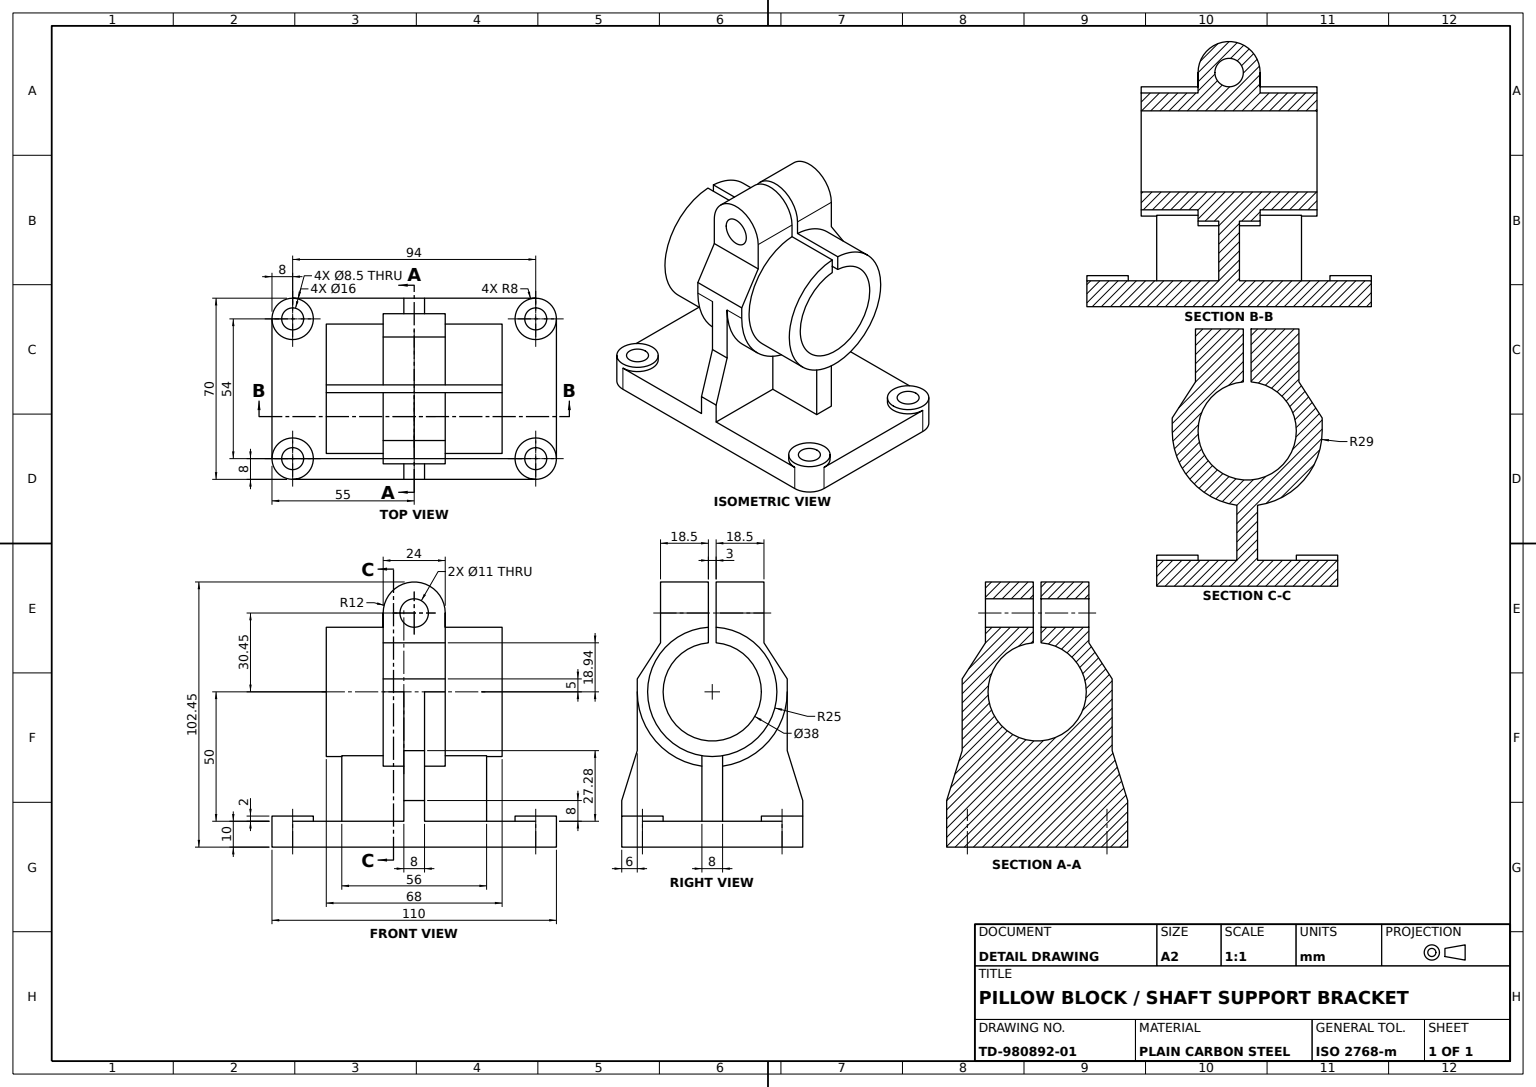
solid
v1 (47,-48,35)
v2 (47,-48,19)
e1 v1 v2 CIRCLE(AX(P(47,-48,27),D(0,1,0),D(0,0,1)),8)
e2 v2 v1 CIRCLE(AX(P(47,-48,27),D(0,1,0),D(0,0,1)),8)
v3 (47,-48,22.75)
v4 (47,-48,31.25)
e3 v3 v4 CIRCLE(AX(P(47,-48,27),D(0,1,0),D(0,0,1)),4.25)
e4 v4 v3 CIRCLE(AX(P(47,-48,27),D(0,1,0),D(0,0,1)),4.25)
face PLANE(AX(P(47,-48,27),D(0,1,0),D(0,0,1))) [e1 e2] [-e3 -e4]
v5 (-34,0,-19)
v6 (-34,0,19)
e5 v5 v6 CIRCLE(AX(P(-34,0,0),D(-1,0,0),D(0,0,1)),19)
v7 (34,0,19)
e6 v7 v6 LINE
v8 (34,0,-19)
e7 v8 v7 CIRCLE(AX(P(34,0,0),D(-1,0,0),D(0,0,1)),19)
e8 v8 v5 LINE
face CYL(AX(P(34,0,0),D(-1,0,0),D(0,0,1)),19) rev [e5 -e6 -e7 e8]
v9 (-12,0,-25)
v10 (-34,0,-25)
e9 v9 v10 LINE
v11 (-34,24.954959,-1.5)
e10 v10 v11 CIRCLE(AX(P(-34,0,0),D(1,0,0),D(0,0,1)),25)
v12 (-12,24.954959,-1.5)
e11 v12 v11 LINE
e12 v12 v9 CIRCLE(AX(P(-12,0,0),D(-1,0,0),D(0,0,1)),25)
face CYL(AX(P(34,0,0),D(-1,0,0),D(0,0,1)),25) [e9 e10 -e11 e12]
v13 (-4,-42,35)
v14 (-4,-50,35)
e13 v13 v14 LINE
v15 (-4,-22.719786,29)
e14 v15 v13 LINE
v16 (-4,0,29)
e15 v16 v15 LINE
v17 (-4,-28.722813,4)
e16 v16 v17 CIRCLE(AX(P(-4,0,0),D(1,0,0),D(0,0,-1)),29)
v18 (-4,-50,4)
e17 v17 v18 LINE
e18 v18 v14 LINE
face PLANE(AX(P(-4,-8.77252,0),D(1,0,0),D(0,0,-1))) rev [-e13 -e14 -e15 e16 e17 e18]
v19 (34,0,25)
v20 (12,0,25)
e19 v19 v20 LINE
v21 (34,24.954959,1.5)
e20 v21 v19 CIRCLE(AX(P(34,0,0),D(1,0,0),D(0,0,1)),25)
v22 (12,24.954959,1.5)
e21 v21 v22 LINE
e22 v20 v22 CIRCLE(AX(P(12,0,0),D(-1,0,0),D(0,0,1)),25)
face CYL(AX(P(34,0,0),D(-1,0,0),D(0,0,1)),25) [-e19 -e20 e21 -e22]
v23 (-4,-42,-35)
v24 (-4,-50,-35)
e23 v23 v24 LINE
v25 (-4,-50,-4)
e24 v24 v25 LINE
v26 (-4,-28.722813,-4)
e25 v25 v26 LINE
v27 (-4,0,-29)
e26 v27 v26 CIRCLE(AX(P(-4,0,0),D(-1,0,0),D(0,0,-1)),29)
v28 (-4,-22.719786,-29)
e27 v27 v28 LINE
e28 v28 v23 LINE
face PLANE(AX(P(-4,-8.77252,0),D(1,0,0),D(0,0,-1))) rev [e23 e24 e25 -e26 e27 e28]
v29 (12,24.954959,-1.5)
v30 (12,30.454959,-1.5)
e29 v29 v30 LINE
v31 (-12,30.454959,-1.5)
e30 v30 v31 CIRCLE(AX(P(0,30.454959,-1.5),D(0,0,1),D(1,0,0)),12)
e31 v31 v12 LINE
v32 (-34,18.940697,-1.5)
e32 v11 v32 LINE
v33 (34,18.940697,-1.5)
e33 v33 v32 LINE
v34 (34,24.954959,-1.5)
e34 v34 v33 LINE
e35 v34 v29 LINE
v35 (5.5,30.454959,-1.5)
v36 (-5.5,30.454959,-1.5)
e36 v35 v36 CIRCLE(AX(P(0,30.454959,-1.5),D(0,0,1),D(1,0,0)),5.5)
e37 v36 v35 CIRCLE(AX(P(0,30.454959,-1.5),D(0,0,1),D(1,0,0)),5.5)
face PLANE(AX(P(34,18.940697,-1.5),D(0,0,-1),D(-1,0,0))) rev [e29 e30 e31 e11 e32 -e33 -e34 e35] [-e36 -e37]
v37 (47,-60,-22.75)
v38 (47,-48,-22.75)
e38 v37 v38 LINE
v39 (47,-60,-31.25)
e39 v39 v37 CIRCLE(AX(P(47,-60,-27),D(0,1,0),D(0,0,-1)),4.25)
v40 (47,-48,-31.25)
e40 v39 v40 LINE
e41 v40 v38 CIRCLE(AX(P(47,-48,-27),D(0,1,0),D(0,0,1)),4.25)
face CYL(AX(P(47,-60.001,-27),D(0,1,0),D(0,0,1)),4.25) rev [-e38 -e39 e40 e41]
v41 (55,-60,27)
v42 (47,-60,35)
e42 v41 v42 CIRCLE(AX(P(47,-60,27),D(0,-1,0),D(0,0,-1)),8)
v43 (55,-50,27)
e43 v41 v43 LINE
v44 (47,-50,19)
e44 v43 v44 CIRCLE(AX(P(47,-50,27),D(0,1,0),D(0,0,1)),8)
e45 v44 v2 LINE
v45 (47,-50,35)
e46 v45 v1 LINE
e47 v42 v45 LINE
face CYL(AX(P(47,-60,27),D(0,1,0),D(0,0,1)),8) [-e42 e43 e44 e45 -e1 -e46 -e47]
v46 (-47,-60,-31.25)
v47 (-47,-48,-31.25)
e48 v46 v47 LINE
v48 (-47,-60,-22.75)
e49 v48 v46 CIRCLE(AX(P(-47,-60,-27),D(0,1,0),D(0,0,-1)),4.25)
v49 (-47,-48,-22.75)
e50 v48 v49 LINE
e51 v49 v47 CIRCLE(AX(P(-47,-48,-27),D(0,1,0),D(0,0,1)),4.25)
face CYL(AX(P(-47,-60.001,-27),D(0,1,0),D(0,0,1)),4.25) rev [-e48 -e49 e50 e51]
v50 (12,-28.722813,4)
v51 (4,-28.722813,4)
e52 v50 v51 LINE
v52 (12,0,29)
e53 v52 v50 CIRCLE(AX(P(12,0,0),D(1,0,0),D(0,0,-1)),29)
v53 (4,0,29)
e54 v52 v53 LINE
e55 v53 v51 CIRCLE(AX(P(4,0,0),D(1,0,0),D(0,0,-1)),29)
face CYL(AX(P(12,0,0),D(-1,0,0),D(0,0,1)),29) [-e52 -e53 e54 e55]
v54 (-12,0,-29)
v55 (-12,-28.722813,-4)
e56 v54 v55 CIRCLE(AX(P(-12,0,0),D(-1,0,0),D(0,0,1)),29)
v56 (-12,-24.677925,-4)
e57 v55 v56 LINE
e58 v9 v56 CIRCLE(AX(P(-12,0,0),D(-1,0,0),D(0,0,1)),25)
v57 (-12,30.454959,-20)
e59 v57 v31 LINE
v58 (-12,18.940697,-20)
e60 v57 v58 LINE
v59 (-12,5,-29)
e61 v58 v59 LINE
e62 v59 v54 LINE
face PLANE(AX(P(-12,30.454959,-20),D(-1,0,0),D(0,0,1))) [e56 e57 -e58 -e12 -e31 -e59 e60 e61 e62]
v60 (-34,24.954959,1.5)
v61 (-34,0,25)
e63 v60 v61 CIRCLE(AX(P(-34,0,0),D(1,0,0),D(0,0,1)),25)
v62 (-12,0,25)
e64 v62 v61 LINE
v63 (-12,24.954959,1.5)
e65 v63 v62 CIRCLE(AX(P(-12,0,0),D(1,0,0),D(0,0,-1)),25)
e66 v63 v60 LINE
face CYL(AX(P(34,0,0),D(-1,0,0),D(0,0,1)),25) [e63 -e64 -e65 e66]
v64 (-47,-60,31.25)
v65 (-47,-48,31.25)
e67 v64 v65 LINE
v66 (-47,-60,22.75)
e68 v66 v64 CIRCLE(AX(P(-47,-60,27),D(0,1,0),D(0,0,-1)),4.25)
v67 (-47,-48,22.75)
e69 v66 v67 LINE
e70 v67 v65 CIRCLE(AX(P(-47,-48,27),D(0,1,0),D(0,0,1)),4.25)
face CYL(AX(P(-47,-60.001,27),D(0,1,0),D(0,0,1)),4.25) rev [-e67 -e68 e69 e70]
v68 (-5.5,30.454959,-20)
e71 v68 v36 LINE
v69 (5.5,30.454959,-20)
e72 v69 v68 CIRCLE(AX(P(0,30.454959,-20),D(0,0,1),D(1,0,0)),5.5)
e73 v69 v35 LINE
face CYL(AX(P(0,30.454959,-20),D(0,0,1),D(1,0,0)),5.5) rev [-e71 -e72 e73 e36]
v70 (47,-50,-35)
v71 (47,-50,-19)
e74 v70 v71 CIRCLE(AX(P(47,-50,-27),D(0,1,0),D(0,0,1)),8)
v72 (47,-48,-19)
e75 v71 v72 LINE
v73 (47,-48,-35)
e76 v73 v72 CIRCLE(AX(P(47,-48,-27),D(0,1,0),D(0,0,1)),8)
e77 v70 v73 LINE
face CYL(AX(P(47,-60,-27),D(0,1,0),D(0,0,1)),8) [e74 e75 -e76 -e77]
v74 (-12,-24.677925,4)
v75 (-28,-24.677925,4)
e78 v74 v75 LINE
v76 (-28,-50,4)
e79 v75 v76 LINE
e80 v18 v76 LINE
v77 (-12,-28.722813,4)
e81 v17 v77 LINE
e82 v77 v74 LINE
face PLANE(AX(P(28,-50,4),D(0,0,-1),D(0,1,0))) rev [e78 e79 -e80 -e17 e81 e82]
v78 (-47,-48,35)
v79 (-47,-48,19)
e83 v78 v79 CIRCLE(AX(P(-47,-48,27),D(0,1,0),D(0,0,1)),8)
v80 (-47,-50,35)
e84 v80 v78 LINE
v81 (-47,-50,19)
e85 v80 v81 CIRCLE(AX(P(-47,-50,27),D(0,1,0),D(0,0,1)),8)
e86 v81 v79 LINE
face CYL(AX(P(-47,-60,27),D(0,1,0),D(0,0,1)),8) [-e83 -e84 e85 e86]
v82 (4,-50,35)
e87 v45 v82 LINE
v83 (4,-42,35)
e88 v83 v82 LINE
e89 v13 v83 LINE
e90 v14 v80 LINE
v84 (-47,-60,35)
e91 v84 v80 LINE
e92 v42 v84 LINE
face PLANE(AX(P(47,-60,35),D(0,0,-1),D(-1,0,0))) rev [e87 -e88 -e89 e13 e90 -e91 -e92 e47]
e93 v46 v48 CIRCLE(AX(P(-47,-60,-27),D(0,1,0),D(0,0,-1)),4.25)
e94 v47 v49 CIRCLE(AX(P(-47,-48,-27),D(0,1,0),D(0,0,1)),4.25)
face CYL(AX(P(-47,-60.001,-27),D(0,1,0),D(0,0,1)),4.25) rev [-e50 -e93 e48 e94]
v85 (4,-22.719786,-29)
e95 v28 v85 LINE
v86 (4,-42,-35)
e96 v85 v86 LINE
e97 v23 v86 LINE
face PLANE(AX(P(0,-22.719786,-29),D(0,-0.297143819,0.954832735),D(0,-0.954832735,-0.297143819))) rev [-e28 e95 e96 -e97]
v87 (34,0,-25)
e98 v19 v87 CIRCLE(AX(P(34,0,0),D(1,0,0),D(0,0,1)),25)
e99 v87 v34 CIRCLE(AX(P(34,0,0),D(1,0,0),D(0,0,1)),25)
e100 v33 v8 CIRCLE(AX(P(34,0,0),D(-1,0,0),D(0,0,1)),19)
v88 (34,18.940697,1.5)
e101 v7 v88 CIRCLE(AX(P(34,0,0),D(-1,0,0),D(0,0,1)),19)
e102 v88 v21 LINE
face PLANE(AX(P(34,0,0),D(-1,0,0),D(0,0,1))) rev [e20 e98 e99 e34 e100 e7 e101 e102]
e103 v44 v45 CIRCLE(AX(P(47,-50,27),D(0,1,0),D(0,0,1)),8)
face CYL(AX(P(47,-60,27),D(0,1,0),D(0,0,1)),8) [-e45 e103 e46 -e2]
v89 (4,-50,-35)
e104 v86 v89 LINE
e105 v89 v70 LINE
v90 (47,-60,-35)
e106 v90 v70 LINE
v91 (-47,-60,-35)
e107 v91 v90 LINE
v92 (-47,-50,-35)
e108 v91 v92 LINE
e109 v92 v24 LINE
face PLANE(AX(P(47,-60,-35),D(0,0,1),D(1,0,0))) rev [e104 e105 -e106 -e107 e108 e109 -e23 e97]
e110 v65 v67 CIRCLE(AX(P(-47,-48,27),D(0,1,0),D(0,0,1)),4.25)
e111 v64 v66 CIRCLE(AX(P(-47,-60,27),D(0,1,0),D(0,0,-1)),4.25)
face CYL(AX(P(-47,-60.001,27),D(0,1,0),D(0,0,1)),4.25) rev [e110 -e69 -e111 e67]
v93 (-28,-24.677925,-4)
e112 v56 v93 LINE
e113 v93 v75 CIRCLE(AX(P(-28,0,0),D(-1,0,0),D(0,0,-1)),25)
e114 v62 v74 CIRCLE(AX(P(-12,0,0),D(1,0,0),D(0,0,-1)),25)
e115 v61 v10 CIRCLE(AX(P(-34,0,0),D(1,0,0),D(0,0,1)),25)
face CYL(AX(P(34,0,0),D(-1,0,0),D(0,0,1)),25) [-e9 e58 e112 e113 -e78 -e114 e64 e115]
e116 v68 v69 CIRCLE(AX(P(0,30.454959,-20),D(0,0,1),D(1,0,0)),5.5)
face CYL(AX(P(0,30.454959,-20),D(0,0,1),D(1,0,0)),5.5) rev [-e73 -e116 e71 e37]
v94 (4,-22.719786,29)
e117 v15 v94 LINE
e118 v94 v83 LINE
face PLANE(AX(P(0,-22.719786,29),D(0,0.297143819,0.954832735),D(0,-0.954832735,0.297143819))) [-e117 e14 e89 -e118]
v95 (12,-28.722813,-4)
v96 (12,-24.677925,-4)
e119 v95 v96 LINE
v97 (12,0,-29)
e120 v97 v95 CIRCLE(AX(P(12,0,0),D(-1,0,0),D(0,0,1)),29)
v98 (12,5,-29)
e121 v98 v97 LINE
v99 (12,18.940697,-20)
e122 v99 v98 LINE
v100 (12,30.454959,-20)
e123 v99 v100 LINE
e124 v100 v30 LINE
v101 (12,0,-25)
e125 v101 v29 CIRCLE(AX(P(12,0,0),D(1,0,0),D(0,0,-1)),25)
e126 v96 v101 CIRCLE(AX(P(12,0,0),D(1,0,0),D(0,0,-1)),25)
face PLANE(AX(P(12,18.940697,-20),D(1,0,0),D(0,0,-1))) [-e119 -e120 -e121 -e122 e123 e124 -e29 -e125 -e126]
e127 v32 v5 CIRCLE(AX(P(-34,0,0),D(-1,0,0),D(0,0,1)),19)
face CYL(AX(P(34,0,0),D(-1,0,0),D(0,0,1)),19) rev [e127 -e8 -e100 e33]
e128 v53 v94 LINE
v102 (12,5,29)
e129 v102 v52 LINE
v103 (-12,5,29)
e130 v102 v103 LINE
v104 (-12,0,29)
e131 v103 v104 LINE
e132 v16 v104 LINE
face PLANE(AX(P(12,5,29),D(0,0,-1),D(-1,0,0))) rev [e117 -e128 -e54 -e129 e130 e131 -e132 e15]
v105 (4,0,-29)
e133 v97 v105 LINE
e134 v105 v85 LINE
e135 v27 v54 LINE
e136 v98 v59 LINE
face PLANE(AX(P(12,5,-29),D(0,0,-1),D(-1,0,0))) [e121 e133 e134 -e95 -e27 e135 -e62 -e136]
e137 v100 v57 CIRCLE(AX(P(0,30.454959,-20),D(0,0,1),D(1,0,0)),12)
face CYL(AX(P(0,30.454959,-20),D(0,0,1),D(1,0,0)),12) [e137 e59 -e30 -e124]
e138 v38 v40 CIRCLE(AX(P(47,-48,-27),D(0,1,0),D(0,0,1)),4.25)
e139 v72 v73 CIRCLE(AX(P(47,-48,-27),D(0,1,0),D(0,0,1)),8)
face PLANE(AX(P(47,-48,-27),D(0,1,0),D(0,0,1))) [-e41 -e138] [e76 e139]
e140 v104 v77 CIRCLE(AX(P(-12,0,0),D(1,0,0),D(0,0,-1)),29)
v106 (-12,18.940697,20)
e141 v106 v103 LINE
v107 (-12,30.454959,20)
e142 v107 v106 LINE
v108 (-12,30.454959,1.5)
e143 v107 v108 LINE
e144 v108 v63 LINE
face PLANE(AX(P(-12,30.454959,20),D(1,0,0),D(0,0,-1))) rev [e114 -e82 -e140 -e131 -e141 -e142 e143 e144 e65]
face CYL(AX(P(12,0,0),D(-1,0,0),D(0,0,1)),29) [-e16 e132 e140 -e81]
v109 (5.5,30.454959,20)
v110 (5.5,30.454959,1.5)
e145 v109 v110 LINE
v111 (-5.5,30.454959,20)
e146 v109 v111 CIRCLE(AX(P(0,30.454959,20),D(0,0,1),D(1,0,0)),5.5)
v112 (-5.5,30.454959,1.5)
e147 v111 v112 LINE
e148 v110 v112 CIRCLE(AX(P(0,30.454959,1.5),D(0,0,1),D(1,0,0)),5.5)
face CYL(AX(P(0,30.454959,20),D(0,0,-1),D(-1,0,0)),5.5) rev [-e145 e146 e147 -e148]
v113 (-47,-50,-19)
e149 v113 v92 CIRCLE(AX(P(-47,-50,-27),D(0,1,0),D(0,0,1)),8)
v114 (-55,-50,-27)
e150 v114 v113 CIRCLE(AX(P(-47,-50,-27),D(0,1,0),D(0,0,1)),8)
v115 (-55,-50,27)
e151 v115 v114 LINE
e152 v81 v115 CIRCLE(AX(P(-47,-50,27),D(0,1,0),D(0,0,1)),8)
v116 (-28,-50,-4)
e153 v76 v116 LINE
e154 v25 v116 LINE
face PLANE(AX(P(47,-50,27),D(0,-1,0),D(0,0,-1))) rev [-e149 -e150 -e151 -e152 -e85 -e90 -e18 e80 e153 -e154 -e24 -e109]
v117 (-34,18.940697,1.5)
e155 v117 v60 LINE
e156 v6 v117 CIRCLE(AX(P(-34,0,0),D(-1,0,0),D(0,0,1)),19)
face PLANE(AX(P(-34,0,0),D(-1,0,0),D(0,0,1))) [-e63 -e155 -e156 -e5 -e127 -e32 -e10 -e115]
e157 v37 v39 CIRCLE(AX(P(47,-60,-27),D(0,1,0),D(0,0,-1)),4.25)
face CYL(AX(P(47,-60.001,-27),D(0,1,0),D(0,0,1)),4.25) rev [-e157 e38 e138 -e40]
e158 v88 v117 LINE
face CYL(AX(P(34,0,0),D(-1,0,0),D(0,0,1)),19) rev [-e158 -e101 e6 e156]
e159 v112 v110 CIRCLE(AX(P(0,30.454959,1.5),D(0,0,1),D(1,0,0)),5.5)
e160 v111 v109 CIRCLE(AX(P(0,30.454959,20),D(0,0,1),D(1,0,0)),5.5)
face CYL(AX(P(0,30.454959,20),D(0,0,-1),D(-1,0,0)),5.5) rev [-e159 -e147 e160 e145]
v118 (28,-24.677925,4)
v119 (12,-24.677925,4)
e161 v118 v119 LINE
v120 (28,-24.677925,-4)
e162 v120 v118 CIRCLE(AX(P(28,0,0),D(-1,0,0),D(0,0,-1)),25)
e163 v120 v96 LINE
e164 v87 v101 LINE
e165 v119 v20 CIRCLE(AX(P(12,0,0),D(-1,0,0),D(0,0,1)),25)
face CYL(AX(P(34,0,0),D(-1,0,0),D(0,0,1)),25) [-e161 -e162 e163 e126 -e164 -e98 e19 -e165]
e166 v79 v78 CIRCLE(AX(P(-47,-48,27),D(0,1,0),D(0,0,1)),8)
v121 (-55,-60,27)
e167 v121 v115 LINE
e168 v84 v121 CIRCLE(AX(P(-47,-60,27),D(0,-1,0),D(0,0,-1)),8)
face CYL(AX(P(-47,-60,27),D(0,1,0),D(0,0,1)),8) [e91 e84 -e166 -e86 e152 -e167 -e168]
e169 v50 v119 LINE
v122 (12,30.454959,1.5)
e170 v22 v122 LINE
v123 (12,30.454959,20)
e171 v123 v122 LINE
v124 (12,18.940697,20)
e172 v124 v123 LINE
e173 v124 v102 LINE
face PLANE(AX(P(12,18.940697,20),D(-1,0,0),D(0,0,1))) rev [e169 e165 e22 e170 -e171 -e172 e173 e129 e53]
v125 (-55,-60,-27)
e174 v125 v91 CIRCLE(AX(P(-47,-60,-27),D(0,-1,0),D(0,0,1)),8)
e175 v125 v114 LINE
v126 (-47,-48,-19)
e176 v113 v126 LINE
v127 (-47,-48,-35)
e177 v127 v126 CIRCLE(AX(P(-47,-48,-27),D(0,1,0),D(0,0,1)),8)
e178 v92 v127 LINE
face CYL(AX(P(-47,-60,-27),D(0,1,0),D(0,0,1)),8) [-e174 e175 e150 e176 -e177 -e178 -e108]
e179 v26 v55 LINE
e180 v116 v93 LINE
face PLANE(AX(P(28,-50,-4),D(0,0,1),D(0,-1,0))) rev [-e179 -e25 e154 e180 -e112 -e57]
v128 (4,-50,4)
e181 v51 v128 LINE
v129 (28,-50,4)
e182 v129 v128 LINE
e183 v118 v129 LINE
face PLANE(AX(P(28,-50,4),D(0,0,-1),D(0,1,0))) rev [e161 -e169 e52 e181 -e182 -e183]
v130 (4,-50,-4)
e184 v89 v130 LINE
v131 (28,-50,-4)
e185 v131 v130 LINE
e186 v129 v131 LINE
e187 v128 v82 LINE
v132 (55,-50,-27)
e188 v132 v43 LINE
e189 v71 v132 CIRCLE(AX(P(47,-50,-27),D(0,1,0),D(0,0,1)),8)
face PLANE(AX(P(47,-50,27),D(0,-1,0),D(0,0,-1))) rev [-e105 e184 -e185 -e186 e182 e187 -e87 -e103 -e44 -e188 -e189 -e74]
v133 (4,-28.722813,-4)
e190 v130 v133 LINE
e191 v95 v133 LINE
e192 v131 v120 LINE
face PLANE(AX(P(28,-50,-4),D(0,0,1),D(0,-1,0))) rev [e185 e190 -e191 e119 -e163 -e192]
e193 v105 v133 CIRCLE(AX(P(4,0,0),D(-1,0,0),D(0,0,-1)),29)
face CYL(AX(P(12,0,0),D(-1,0,0),D(0,0,1)),29) [-e193 -e133 e120 e191]
face PLANE(AX(P(28,0,0),D(1,0,0),D(0,0,-1))) [e162 e183 e186 e192]
e194 v122 v108 CIRCLE(AX(P(0,30.454959,1.5),D(0,0,1),D(1,0,0)),12)
face PLANE(AX(P(34,18.940697,1.5),D(0,0,1),D(1,0,0))) rev [e158 e155 -e66 -e144 -e194 -e170 -e21 -e102] [e159 e148]
e195 v126 v127 CIRCLE(AX(P(-47,-48,-27),D(0,1,0),D(0,0,1)),8)
face PLANE(AX(P(-47,-48,-27),D(0,1,0),D(0,0,1))) [e195 e177] [-e51 -e94]
face PLANE(AX(P(-47,-48,27),D(0,1,0),D(0,0,1))) [e83 e166] [-e70 -e110]
e196 v121 v125 LINE
face PLANE(AX(P(-55,-60,-27),D(1,0,0),D(0,0,-1))) rev [-e196 e167 e151 -e175]
e197 v106 v124 LINE
face PLANE(AX(P(12,18.940697,20),D(0,-0.542382246,-0.840131834),D(0,0.840131834,-0.542382246))) rev [-e197 e141 -e130 -e173]
face CYL(AX(P(-47,-60,-27),D(0,1,0),D(0,0,1)),8) [-e195 -e176 e149 e178]
face PLANE(AX(P(-28,0,0),D(1,0,0),D(0,0,-1))) rev [-e153 -e79 -e113 -e180]
v134 (47,-60,31.25)
e198 v134 v4 LINE
v135 (47,-60,22.75)
e199 v135 v3 LINE
e200 v134 v135 CIRCLE(AX(P(47,-60,27),D(0,1,0),D(0,0,-1)),4.25)
face CYL(AX(P(47,-60.001,27),D(0,1,0),D(0,0,1)),4.25) rev [e198 e4 -e199 -e200]
e201 v135 v134 CIRCLE(AX(P(47,-60,27),D(0,1,0),D(0,0,-1)),4.25)
face CYL(AX(P(47,-60.001,27),D(0,1,0),D(0,0,1)),4.25) rev [-e198 -e201 e199 e3]
e202 v123 v107 CIRCLE(AX(P(0,30.454959,20),D(0,0,1),D(1,0,0)),12)
face PLANE(AX(P(0,30.454959,20),D(0,0,1),D(1,0,0))) [e202 e142 e197 e172] [-e160 -e146]
face CYL(AX(P(34,0,0),D(-1,0,0),D(0,0,1)),25) [-e99 e164 e125 -e35]
face PLANE(AX(P(4,-8.77252,0),D(1,0,0),D(0,0,-1))) [e88 -e187 -e181 -e55 e128 e118]
v136 (55,-60,-27)
e203 v136 v41 LINE
e204 v136 v132 LINE
face PLANE(AX(P(55,-60,-27),D(-1,0,0),D(0,0,1))) rev [-e203 e204 e188 -e43]
e205 v58 v99 LINE
face PLANE(AX(P(0,30.454959,-20),D(0,0,-1),D(1,0,0))) [-e123 -e205 -e60 -e137] [e116 e72]
face CYL(AX(P(12,0,0),D(-1,0,0),D(0,0,1)),29) [e26 e179 -e56 -e135]
face CYL(AX(P(0,30.454959,20),D(0,0,-1),D(-1,0,0)),12) [e171 e194 -e143 -e202]
face PLANE(AX(P(12,18.940697,-20),D(0,0.542382246,-0.840131834),D(0,0.840131834,0.542382246))) [-e61 e205 e122 e136]
face PLANE(AX(P(4,-8.77252,0),D(1,0,0),D(0,0,-1))) [e193 -e190 -e184 -e104 -e96 -e134]
e206 v90 v136 CIRCLE(AX(P(47,-60,-27),D(0,-1,0),D(0,0,-1)),8)
face PLANE(AX(P(47,-60,27),D(0,-1,0),D(0,0,-1))) [e157 e39] [e68 e111] [e107 e206 e203 e42 e92 e168 e196 e174] [e49 e93] [e201 e200]
face CYL(AX(P(47,-60,-27),D(0,1,0),D(0,0,1)),8) [e189 -e204 -e206 e106 e77 -e139 -e75]
